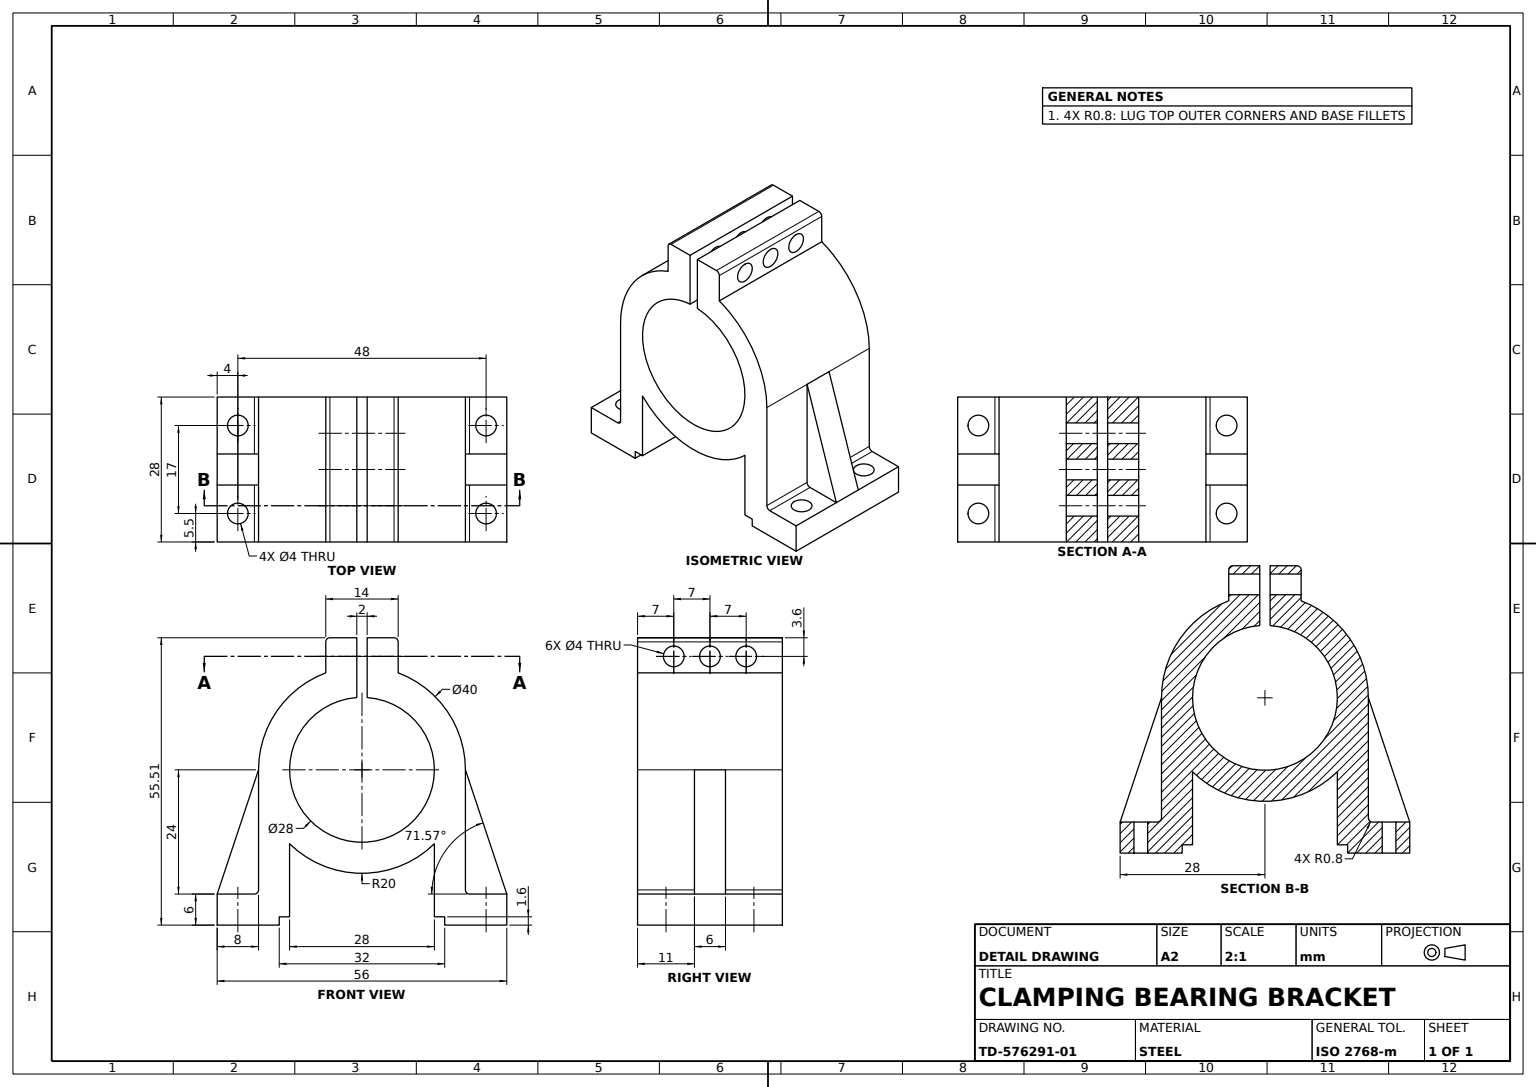
ISO-10303-21;
HEADER;
FILE_DESCRIPTION((''),'2;1');
FILE_NAME('','',(''),(''),'','','');
FILE_SCHEMA(('AUTOMOTIVE_DESIGN'));
ENDSEC;
DATA;
#1=APPLICATION_CONTEXT('');
#2=PRODUCT_CONTEXT('',#1,'mechanical');
#3=PRODUCT('','','',(#2));
#4=PRODUCT_DEFINITION_FORMATION('','',#3);
#5=PRODUCT_DEFINITION_CONTEXT('',#1,'design');
#6=PRODUCT_DEFINITION('','',#4,#5);
#7=PRODUCT_DEFINITION_SHAPE('','',#6);
#8=(LENGTH_UNIT()NAMED_UNIT(*)SI_UNIT(.MILLI.,.METRE.));
#9=(NAMED_UNIT(*)PLANE_ANGLE_UNIT()SI_UNIT($,.RADIAN.));
#10=(NAMED_UNIT(*)SI_UNIT($,.STERADIAN.)SOLID_ANGLE_UNIT());
#11=UNCERTAINTY_MEASURE_WITH_UNIT(LENGTH_MEASURE(0.005),#8,'distance_accuracy_value','');
#12=(GEOMETRIC_REPRESENTATION_CONTEXT(3)GLOBAL_UNCERTAINTY_ASSIGNED_CONTEXT((#11))GLOBAL_UNIT_ASSIGNED_CONTEXT((#8,#9,#10))REPRESENTATION_CONTEXT('',''));
#13=CARTESIAN_POINT('',(22.,-8.5,-24.));
#14=VERTEX_POINT('',#13);
#15=CARTESIAN_POINT('',(24.,-8.5,-24.));
#16=DIRECTION('',(0.,0.,-1.));
#17=DIRECTION('',(-1.,0.,0.));
#18=AXIS2_PLACEMENT_3D('',#15,#16,#17);
#19=CIRCLE('',#18,2.);
#20=EDGE_CURVE('',#14,#14,#19,.T.);
#21=ORIENTED_EDGE('',*,*,#20,.F.);
#22=EDGE_LOOP('',(#21));
#23=FACE_BOUND('',#22,.T.);
#24=CARTESIAN_POINT('',(22.,-8.5,-30.));
#25=VERTEX_POINT('',#24);
#26=CARTESIAN_POINT('',(24.,-8.5,-30.));
#27=AXIS2_PLACEMENT_3D('',#26,#16,#17);
#28=CIRCLE('',#27,2.);
#29=EDGE_CURVE('',#25,#25,#28,.T.);
#30=ORIENTED_EDGE('',*,*,#29,.T.);
#31=EDGE_LOOP('',(#30));
#32=FACE_BOUND('',#31,.T.);
#33=CYLINDRICAL_SURFACE('',#18,2.);
#34=ADVANCED_FACE('',(#23,#32),#33,.F.);
#35=CARTESIAN_POINT('',(-22.,-8.5,-30.));
#36=VERTEX_POINT('',#35);
#37=CARTESIAN_POINT('',(-24.,-8.5,-30.));
#38=DIRECTION('',(0.,0.,1.));
#39=DIRECTION('',(1.,0.,0.));
#40=AXIS2_PLACEMENT_3D('',#37,#38,#39);
#41=CIRCLE('',#40,2.);
#42=EDGE_CURVE('',#36,#36,#41,.T.);
#43=ORIENTED_EDGE('',*,*,#42,.F.);
#44=EDGE_LOOP('',(#43));
#45=FACE_BOUND('',#44,.T.);
#46=CARTESIAN_POINT('',(-26.,-8.5,-24.));
#47=VERTEX_POINT('',#46);
#48=CARTESIAN_POINT('',(-24.,-8.5,-24.));
#49=AXIS2_PLACEMENT_3D('',#48,#16,#17);
#50=CIRCLE('',#49,2.);
#51=EDGE_CURVE('',#47,#47,#50,.T.);
#52=ORIENTED_EDGE('',*,*,#51,.F.);
#53=EDGE_LOOP('',(#52));
#54=FACE_BOUND('',#53,.T.);
#55=CYLINDRICAL_SURFACE('',#49,2.);
#56=ADVANCED_FACE('',(#45,#54),#55,.F.);
#57=CARTESIAN_POINT('',(-26.,8.5,-24.));
#58=VERTEX_POINT('',#57);
#59=CARTESIAN_POINT('',(-24.,8.5,-24.));
#60=AXIS2_PLACEMENT_3D('',#59,#16,#17);
#61=CIRCLE('',#60,2.);
#62=EDGE_CURVE('',#58,#58,#61,.T.);
#63=ORIENTED_EDGE('',*,*,#62,.F.);
#64=EDGE_LOOP('',(#63));
#65=FACE_BOUND('',#64,.T.);
#66=CARTESIAN_POINT('',(-22.,8.5,-30.));
#67=VERTEX_POINT('',#66);
#68=CARTESIAN_POINT('',(-24.,8.5,-30.));
#69=AXIS2_PLACEMENT_3D('',#68,#38,#39);
#70=CIRCLE('',#69,2.);
#71=EDGE_CURVE('',#67,#67,#70,.T.);
#72=ORIENTED_EDGE('',*,*,#71,.F.);
#73=EDGE_LOOP('',(#72));
#74=FACE_BOUND('',#73,.T.);
#75=CYLINDRICAL_SURFACE('',#60,2.);
#76=ADVANCED_FACE('',(#65,#74),#75,.F.);
#77=CARTESIAN_POINT('',(22.,8.5,-30.));
#78=VERTEX_POINT('',#77);
#79=CARTESIAN_POINT('',(24.,8.5,-30.));
#80=AXIS2_PLACEMENT_3D('',#79,#16,#17);
#81=CIRCLE('',#80,2.);
#82=EDGE_CURVE('',#78,#78,#81,.T.);
#83=ORIENTED_EDGE('',*,*,#82,.T.);
#84=EDGE_LOOP('',(#83));
#85=FACE_BOUND('',#84,.T.);
#86=CARTESIAN_POINT('',(22.,8.5,-24.));
#87=VERTEX_POINT('',#86);
#88=CARTESIAN_POINT('',(24.,8.5,-24.));
#89=AXIS2_PLACEMENT_3D('',#88,#16,#17);
#90=CIRCLE('',#89,2.);
#91=EDGE_CURVE('',#87,#87,#90,.T.);
#92=ORIENTED_EDGE('',*,*,#91,.F.);
#93=EDGE_LOOP('',(#92));
#94=FACE_BOUND('',#93,.T.);
#95=CYLINDRICAL_SURFACE('',#89,2.);
#96=ADVANCED_FACE('',(#85,#94),#95,.F.);
#97=CARTESIAN_POINT('',(-7.,7.,23.914709));
#98=VERTEX_POINT('',#97);
#99=CARTESIAN_POINT('',(-7.,7.,21.914709));
#100=AXIS2_PLACEMENT_3D('',#99,#17,#38);
#101=CIRCLE('',#100,2.);
#102=EDGE_CURVE('',#98,#98,#101,.T.);
#103=ORIENTED_EDGE('',*,*,#102,.F.);
#104=EDGE_LOOP('',(#103));
#105=FACE_BOUND('',#104,.T.);
#106=CARTESIAN_POINT('',(-7.,-7.,23.914709));
#107=VERTEX_POINT('',#106);
#108=CARTESIAN_POINT('',(-7.,-7.,21.914709));
#109=AXIS2_PLACEMENT_3D('',#108,#17,#38);
#110=CIRCLE('',#109,2.);
#111=EDGE_CURVE('',#107,#107,#110,.T.);
#112=ORIENTED_EDGE('',*,*,#111,.F.);
#113=EDGE_LOOP('',(#112));
#114=FACE_BOUND('',#113,.T.);
#115=CARTESIAN_POINT('',(-7.,-14.,24.714709));
#116=VERTEX_POINT('',#115);
#117=CARTESIAN_POINT('',(-7.,14.,24.714709));
#118=VERTEX_POINT('',#117);
#119=DIRECTION('',(0.,1.,0.));
#120=VECTOR('',#119,1000.);
#121=LINE('',#115,#120);
#122=EDGE_CURVE('',#116,#118,#121,.T.);
#123=ORIENTED_EDGE('',*,*,#122,.T.);
#124=CARTESIAN_POINT('',(-7.,14.,18.734994));
#125=VERTEX_POINT('',#124);
#126=CARTESIAN_POINT('',(-7.,14.,18.314709));
#127=VECTOR('',#38,1000.);
#128=LINE('',#126,#127);
#129=EDGE_CURVE('',#125,#118,#128,.T.);
#130=ORIENTED_EDGE('',*,*,#129,.F.);
#131=CARTESIAN_POINT('',(-7.,-14.,18.734994));
#132=VERTEX_POINT('',#131);
#133=LINE('',#131,#120);
#134=EDGE_CURVE('',#132,#125,#133,.T.);
#135=ORIENTED_EDGE('',*,*,#134,.F.);
#136=CARTESIAN_POINT('',(-7.,-14.,18.314709));
#137=LINE('',#136,#127);
#138=EDGE_CURVE('',#132,#116,#137,.T.);
#139=ORIENTED_EDGE('',*,*,#138,.T.);
#140=EDGE_LOOP('',(#123,#130,#135,#139));
#141=FACE_BOUND('',#140,.T.);
#142=CARTESIAN_POINT('',(-7.,0.,23.914709));
#143=VERTEX_POINT('',#142);
#144=CARTESIAN_POINT('',(-7.,0.,21.914709));
#145=AXIS2_PLACEMENT_3D('',#144,#17,#38);
#146=CIRCLE('',#145,2.);
#147=EDGE_CURVE('',#143,#143,#146,.T.);
#148=ORIENTED_EDGE('',*,*,#147,.F.);
#149=EDGE_LOOP('',(#148));
#150=FACE_BOUND('',#149,.T.);
#151=AXIS2_PLACEMENT_3D('',#136,#17,#38);
#152=PLANE('',#151);
#153=ADVANCED_FACE('',(#105,#114,#141,#150),#152,.T.);
#154=CARTESIAN_POINT('',(20.,3.,0.));
#155=VERTEX_POINT('',#154);
#156=CARTESIAN_POINT('',(20.,3.,-23.2));
#157=VERTEX_POINT('',#156);
#158=VECTOR('',#16,1000.);
#159=LINE('',#154,#158);
#160=EDGE_CURVE('',#155,#157,#159,.T.);
#161=ORIENTED_EDGE('',*,*,#160,.F.);
#162=CARTESIAN_POINT('',(28.,3.,-24.));
#163=VERTEX_POINT('',#162);
#164=DIRECTION('',(-0.316227766,0.,0.948683298));
#165=VECTOR('',#164,1000.);
#166=LINE('',#162,#165);
#167=EDGE_CURVE('',#163,#155,#166,.T.);
#168=ORIENTED_EDGE('',*,*,#167,.F.);
#169=CARTESIAN_POINT('',(20.8,3.,-24.));
#170=VERTEX_POINT('',#169);
#171=CARTESIAN_POINT('',(20.,3.,-24.));
#172=VECTOR('',#39,1000.);
#173=LINE('',#171,#172);
#174=EDGE_CURVE('',#170,#163,#173,.T.);
#175=ORIENTED_EDGE('',*,*,#174,.F.);
#176=CARTESIAN_POINT('',(20.8,3.,-23.2));
#177=AXIS2_PLACEMENT_3D('',#176,#119,#38);
#178=CIRCLE('',#177,0.8);
#179=EDGE_CURVE('',#170,#157,#178,.T.);
#180=ORIENTED_EDGE('',*,*,#179,.T.);
#181=EDGE_LOOP('',(#161,#168,#175,#180));
#182=FACE_BOUND('',#181,.T.);
#183=CARTESIAN_POINT('',(0.,3.,0.));
#184=AXIS2_PLACEMENT_3D('',#183,#119,#38);
#185=PLANE('',#184);
#186=ADVANCED_FACE('',(#182),#185,.T.);
#187=CARTESIAN_POINT('',(-20.8,3.,-24.));
#188=VERTEX_POINT('',#187);
#189=CARTESIAN_POINT('',(-28.,3.,-24.));
#190=VERTEX_POINT('',#189);
#191=CARTESIAN_POINT('',(-20.,3.,-24.));
#192=VECTOR('',#17,1000.);
#193=LINE('',#191,#192);
#194=EDGE_CURVE('',#188,#190,#193,.T.);
#195=ORIENTED_EDGE('',*,*,#194,.F.);
#196=CARTESIAN_POINT('',(-20.8,14.,-24.));
#197=VERTEX_POINT('',#196);
#198=CARTESIAN_POINT('',(-20.8,0.,-24.));
#199=DIRECTION('',(0.,-1.,0.));
#200=VECTOR('',#199,1000.);
#201=LINE('',#198,#200);
#202=EDGE_CURVE('',#188,#197,#201,.F.);
#203=ORIENTED_EDGE('',*,*,#202,.T.);
#204=CARTESIAN_POINT('',(-28.,14.,-24.));
#205=VERTEX_POINT('',#204);
#206=CARTESIAN_POINT('',(-14.,14.,-24.));
#207=LINE('',#206,#192);
#208=EDGE_CURVE('',#197,#205,#207,.T.);
#209=ORIENTED_EDGE('',*,*,#208,.T.);
#210=LINE('',#204,#200);
#211=EDGE_CURVE('',#205,#190,#210,.T.);
#212=ORIENTED_EDGE('',*,*,#211,.T.);
#213=EDGE_LOOP('',(#195,#203,#209,#212));
#214=FACE_BOUND('',#213,.T.);
#215=ORIENTED_EDGE('',*,*,#62,.T.);
#216=EDGE_LOOP('',(#215));
#217=FACE_BOUND('',#216,.T.);
#218=CARTESIAN_POINT('',(0.,0.,-24.));
#219=AXIS2_PLACEMENT_3D('',#218,#38,#39);
#220=PLANE('',#219);
#221=ADVANCED_FACE('',(#214,#217),#220,.T.);
#222=CARTESIAN_POINT('',(-28.,14.,-30.));
#223=VERTEX_POINT('',#222);
#224=LINE('',#222,#127);
#225=EDGE_CURVE('',#223,#205,#224,.T.);
#226=ORIENTED_EDGE('',*,*,#225,.F.);
#227=CARTESIAN_POINT('',(-28.,-14.,-30.));
#228=VERTEX_POINT('',#227);
#229=LINE('',#222,#200);
#230=EDGE_CURVE('',#223,#228,#229,.T.);
#231=ORIENTED_EDGE('',*,*,#230,.T.);
#232=CARTESIAN_POINT('',(-28.,-14.,-24.));
#233=VERTEX_POINT('',#232);
#234=LINE('',#227,#127);
#235=EDGE_CURVE('',#228,#233,#234,.T.);
#236=ORIENTED_EDGE('',*,*,#235,.T.);
#237=CARTESIAN_POINT('',(-28.,-3.,-24.));
#238=VERTEX_POINT('',#237);
#239=EDGE_CURVE('',#238,#233,#210,.T.);
#240=ORIENTED_EDGE('',*,*,#239,.F.);
#241=LINE('',#237,#120);
#242=EDGE_CURVE('',#238,#190,#241,.T.);
#243=ORIENTED_EDGE('',*,*,#242,.T.);
#244=ORIENTED_EDGE('',*,*,#211,.F.);
#245=EDGE_LOOP('',(#226,#231,#236,#240,#243,#244));
#246=FACE_BOUND('',#245,.T.);
#247=AXIS2_PLACEMENT_3D('',#222,#17,#38);
#248=PLANE('',#247);
#249=ADVANCED_FACE('',(#246),#248,.T.);
#250=CARTESIAN_POINT('',(-20.,-3.,0.));
#251=VERTEX_POINT('',#250);
#252=DIRECTION('',(0.316227766,0.,0.948683298));
#253=VECTOR('',#252,1000.);
#254=LINE('',#237,#253);
#255=EDGE_CURVE('',#238,#251,#254,.T.);
#256=ORIENTED_EDGE('',*,*,#255,.T.);
#257=CARTESIAN_POINT('',(-20.,3.,0.));
#258=VERTEX_POINT('',#257);
#259=LINE('',#250,#120);
#260=EDGE_CURVE('',#251,#258,#259,.T.);
#261=ORIENTED_EDGE('',*,*,#260,.T.);
#262=LINE('',#189,#253);
#263=EDGE_CURVE('',#190,#258,#262,.T.);
#264=ORIENTED_EDGE('',*,*,#263,.F.);
#265=ORIENTED_EDGE('',*,*,#242,.F.);
#266=EDGE_LOOP('',(#256,#261,#264,#265));
#267=FACE_BOUND('',#266,.T.);
#268=DIRECTION('',(-0.948683298,0.,0.316227766));
#269=AXIS2_PLACEMENT_3D('',#237,#268,#252);
#270=PLANE('',#269);
#271=ADVANCED_FACE('',(#267),#270,.T.);
#272=CARTESIAN_POINT('',(7.,-14.,24.714709));
#273=VERTEX_POINT('',#272);
#274=CARTESIAN_POINT('',(6.2,-14.,25.514709));
#275=VERTEX_POINT('',#274);
#276=CARTESIAN_POINT('',(6.2,-14.,24.714709));
#277=AXIS2_PLACEMENT_3D('',#276,#199,#16);
#278=CIRCLE('',#277,0.8);
#279=EDGE_CURVE('',#273,#275,#278,.T.);
#280=ORIENTED_EDGE('',*,*,#279,.F.);
#281=CARTESIAN_POINT('',(7.,14.,24.714709));
#282=VERTEX_POINT('',#281);
#283=LINE('',#272,#120);
#284=EDGE_CURVE('',#282,#273,#283,.F.);
#285=ORIENTED_EDGE('',*,*,#284,.F.);
#286=CARTESIAN_POINT('',(6.2,14.,25.514709));
#287=VERTEX_POINT('',#286);
#288=CARTESIAN_POINT('',(6.2,14.,24.714709));
#289=AXIS2_PLACEMENT_3D('',#288,#199,#16);
#290=CIRCLE('',#289,0.8);
#291=EDGE_CURVE('',#287,#282,#290,.F.);
#292=ORIENTED_EDGE('',*,*,#291,.F.);
#293=LINE('',#274,#120);
#294=EDGE_CURVE('',#275,#287,#293,.T.);
#295=ORIENTED_EDGE('',*,*,#294,.F.);
#296=EDGE_LOOP('',(#280,#285,#292,#295));
#297=FACE_BOUND('',#296,.T.);
#298=AXIS2_PLACEMENT_3D('',#276,#119,#38);
#299=CYLINDRICAL_SURFACE('',#298,0.8);
#300=ADVANCED_FACE('',(#297),#299,.T.);
#301=ORIENTED_EDGE('',*,*,#82,.F.);
#302=EDGE_LOOP('',(#301));
#303=FACE_BOUND('',#302,.T.);
#304=CARTESIAN_POINT('',(16.,-14.,-30.));
#305=VERTEX_POINT('',#304);
#306=CARTESIAN_POINT('',(16.,14.,-30.));
#307=VERTEX_POINT('',#306);
#308=CARTESIAN_POINT('',(16.,-16.,-30.));
#309=LINE('',#308,#120);
#310=EDGE_CURVE('',#305,#307,#309,.T.);
#311=ORIENTED_EDGE('',*,*,#310,.T.);
#312=CARTESIAN_POINT('',(28.,14.,-30.));
#313=VERTEX_POINT('',#312);
#314=CARTESIAN_POINT('',(14.,14.,-30.));
#315=LINE('',#314,#172);
#316=EDGE_CURVE('',#307,#313,#315,.T.);
#317=ORIENTED_EDGE('',*,*,#316,.T.);
#318=CARTESIAN_POINT('',(28.,-14.,-30.));
#319=VERTEX_POINT('',#318);
#320=LINE('',#312,#200);
#321=EDGE_CURVE('',#313,#319,#320,.T.);
#322=ORIENTED_EDGE('',*,*,#321,.T.);
#323=LINE('',#318,#192);
#324=EDGE_CURVE('',#319,#305,#323,.T.);
#325=ORIENTED_EDGE('',*,*,#324,.T.);
#326=EDGE_LOOP('',(#311,#317,#322,#325));
#327=FACE_BOUND('',#326,.T.);
#328=ORIENTED_EDGE('',*,*,#29,.F.);
#329=EDGE_LOOP('',(#328));
#330=FACE_BOUND('',#329,.T.);
#331=CARTESIAN_POINT('',(0.,0.,-30.));
#332=AXIS2_PLACEMENT_3D('',#331,#16,#17);
#333=PLANE('',#332);
#334=ADVANCED_FACE('',(#303,#327,#330),#333,.T.);
#335=CARTESIAN_POINT('',(20.8,-3.,-24.));
#336=VERTEX_POINT('',#335);
#337=CARTESIAN_POINT('',(28.,-3.,-24.));
#338=VERTEX_POINT('',#337);
#339=CARTESIAN_POINT('',(20.,-3.,-24.));
#340=LINE('',#339,#172);
#341=EDGE_CURVE('',#336,#338,#340,.T.);
#342=ORIENTED_EDGE('',*,*,#341,.T.);
#343=CARTESIAN_POINT('',(20.,-3.,0.));
#344=VERTEX_POINT('',#343);
#345=LINE('',#337,#165);
#346=EDGE_CURVE('',#338,#344,#345,.T.);
#347=ORIENTED_EDGE('',*,*,#346,.T.);
#348=CARTESIAN_POINT('',(20.,-3.,-23.2));
#349=VERTEX_POINT('',#348);
#350=LINE('',#343,#158);
#351=EDGE_CURVE('',#344,#349,#350,.T.);
#352=ORIENTED_EDGE('',*,*,#351,.T.);
#353=CARTESIAN_POINT('',(20.8,-3.,-23.2));
#354=AXIS2_PLACEMENT_3D('',#353,#119,#38);
#355=CIRCLE('',#354,0.8);
#356=EDGE_CURVE('',#349,#336,#355,.F.);
#357=ORIENTED_EDGE('',*,*,#356,.T.);
#358=EDGE_LOOP('',(#342,#347,#352,#357));
#359=FACE_BOUND('',#358,.T.);
#360=CARTESIAN_POINT('',(0.,-3.,0.));
#361=AXIS2_PLACEMENT_3D('',#360,#119,#38);
#362=PLANE('',#361);
#363=ADVANCED_FACE('',(#359),#362,.F.);
#364=CARTESIAN_POINT('',(1.,7.,23.914709));
#365=VERTEX_POINT('',#364);
#366=CARTESIAN_POINT('',(1.,7.,21.914709));
#367=AXIS2_PLACEMENT_3D('',#366,#17,#38);
#368=CIRCLE('',#367,2.);
#369=EDGE_CURVE('',#365,#365,#368,.T.);
#370=ORIENTED_EDGE('',*,*,#369,.F.);
#371=EDGE_LOOP('',(#370));
#372=FACE_BOUND('',#371,.T.);
#373=CARTESIAN_POINT('',(1.,0.,23.914709));
#374=VERTEX_POINT('',#373);
#375=CARTESIAN_POINT('',(1.,0.,21.914709));
#376=AXIS2_PLACEMENT_3D('',#375,#17,#38);
#377=CIRCLE('',#376,2.);
#378=EDGE_CURVE('',#374,#374,#377,.T.);
#379=ORIENTED_EDGE('',*,*,#378,.F.);
#380=EDGE_LOOP('',(#379));
#381=FACE_BOUND('',#380,.T.);
#382=CARTESIAN_POINT('',(1.,-7.,23.914709));
#383=VERTEX_POINT('',#382);
#384=CARTESIAN_POINT('',(1.,-7.,21.914709));
#385=AXIS2_PLACEMENT_3D('',#384,#17,#38);
#386=CIRCLE('',#385,2.);
#387=EDGE_CURVE('',#383,#383,#386,.T.);
#388=ORIENTED_EDGE('',*,*,#387,.F.);
#389=EDGE_LOOP('',(#388));
#390=FACE_BOUND('',#389,.T.);
#391=CARTESIAN_POINT('',(1.,14.,25.514709));
#392=VERTEX_POINT('',#391);
#393=CARTESIAN_POINT('',(1.,-14.,25.514709));
#394=VERTEX_POINT('',#393);
#395=LINE('',#393,#200);
#396=EDGE_CURVE('',#392,#394,#395,.T.);
#397=ORIENTED_EDGE('',*,*,#396,.F.);
#398=CARTESIAN_POINT('',(1.,14.,13.96424));
#399=VERTEX_POINT('',#398);
#400=CARTESIAN_POINT('',(1.,14.,0.));
#401=LINE('',#400,#158);
#402=EDGE_CURVE('',#392,#399,#401,.T.);
#403=ORIENTED_EDGE('',*,*,#402,.T.);
#404=CARTESIAN_POINT('',(1.,-14.,13.96424));
#405=VERTEX_POINT('',#404);
#406=LINE('',#404,#120);
#407=EDGE_CURVE('',#399,#405,#406,.F.);
#408=ORIENTED_EDGE('',*,*,#407,.T.);
#409=CARTESIAN_POINT('',(1.,-14.,0.));
#410=LINE('',#409,#158);
#411=EDGE_CURVE('',#394,#405,#410,.T.);
#412=ORIENTED_EDGE('',*,*,#411,.F.);
#413=EDGE_LOOP('',(#397,#403,#408,#412));
#414=FACE_BOUND('',#413,.T.);
#415=CARTESIAN_POINT('',(1.,-17.5,12.763345));
#416=AXIS2_PLACEMENT_3D('',#415,#17,#38);
#417=PLANE('',#416);
#418=ADVANCED_FACE('',(#372,#381,#390,#414),#417,.T.);
#419=LINE('',#343,#120);
#420=EDGE_CURVE('',#344,#155,#419,.T.);
#421=ORIENTED_EDGE('',*,*,#420,.F.);
#422=ORIENTED_EDGE('',*,*,#346,.F.);
#423=LINE('',#337,#120);
#424=EDGE_CURVE('',#338,#163,#423,.T.);
#425=ORIENTED_EDGE('',*,*,#424,.T.);
#426=ORIENTED_EDGE('',*,*,#167,.T.);
#427=EDGE_LOOP('',(#421,#422,#425,#426));
#428=FACE_BOUND('',#427,.T.);
#429=DIRECTION('',(-0.948683298,0.,-0.316227766));
#430=AXIS2_PLACEMENT_3D('',#337,#429,#164);
#431=PLANE('',#430);
#432=ADVANCED_FACE('',(#428),#431,.F.);
#433=CARTESIAN_POINT('',(-6.2,14.,25.514709));
#434=VERTEX_POINT('',#433);
#435=CARTESIAN_POINT('',(-6.2,14.,24.714709));
#436=AXIS2_PLACEMENT_3D('',#435,#199,#16);
#437=CIRCLE('',#436,0.8);
#438=EDGE_CURVE('',#118,#434,#437,.F.);
#439=ORIENTED_EDGE('',*,*,#438,.F.);
#440=ORIENTED_EDGE('',*,*,#122,.F.);
#441=CARTESIAN_POINT('',(-6.2,-14.,25.514709));
#442=VERTEX_POINT('',#441);
#443=CARTESIAN_POINT('',(-6.2,-14.,24.714709));
#444=AXIS2_PLACEMENT_3D('',#443,#199,#16);
#445=CIRCLE('',#444,0.8);
#446=EDGE_CURVE('',#442,#116,#445,.T.);
#447=ORIENTED_EDGE('',*,*,#446,.F.);
#448=LINE('',#441,#120);
#449=EDGE_CURVE('',#434,#442,#448,.F.);
#450=ORIENTED_EDGE('',*,*,#449,.F.);
#451=EDGE_LOOP('',(#439,#440,#447,#450));
#452=FACE_BOUND('',#451,.T.);
#453=AXIS2_PLACEMENT_3D('',#443,#119,#38);
#454=CYLINDRICAL_SURFACE('',#453,0.8);
#455=ADVANCED_FACE('',(#452),#454,.T.);
#456=ORIENTED_EDGE('',*,*,#20,.T.);
#457=EDGE_LOOP('',(#456));
#458=FACE_BOUND('',#457,.T.);
#459=ORIENTED_EDGE('',*,*,#341,.F.);
#460=CARTESIAN_POINT('',(20.8,-14.,-24.));
#461=VERTEX_POINT('',#460);
#462=LINE('',#460,#200);
#463=EDGE_CURVE('',#336,#461,#462,.T.);
#464=ORIENTED_EDGE('',*,*,#463,.T.);
#465=CARTESIAN_POINT('',(28.,-14.,-24.));
#466=VERTEX_POINT('',#465);
#467=LINE('',#465,#192);
#468=EDGE_CURVE('',#466,#461,#467,.T.);
#469=ORIENTED_EDGE('',*,*,#468,.F.);
#470=CARTESIAN_POINT('',(28.,14.,-24.));
#471=LINE('',#470,#200);
#472=EDGE_CURVE('',#338,#466,#471,.T.);
#473=ORIENTED_EDGE('',*,*,#472,.F.);
#474=EDGE_LOOP('',(#459,#464,#469,#473));
#475=FACE_BOUND('',#474,.T.);
#476=AXIS2_PLACEMENT_3D('',#218,#16,#17);
#477=PLANE('',#476);
#478=ADVANCED_FACE('',(#458,#475),#477,.F.);
#479=CARTESIAN_POINT('',(-1.,0.,19.914709));
#480=VERTEX_POINT('',#479);
#481=CARTESIAN_POINT('',(-1.,0.,21.914709));
#482=AXIS2_PLACEMENT_3D('',#481,#39,#16);
#483=CIRCLE('',#482,2.);
#484=EDGE_CURVE('',#480,#480,#483,.T.);
#485=ORIENTED_EDGE('',*,*,#484,.T.);
#486=EDGE_LOOP('',(#485));
#487=FACE_BOUND('',#486,.T.);
#488=ORIENTED_EDGE('',*,*,#147,.T.);
#489=EDGE_LOOP('',(#488));
#490=FACE_BOUND('',#489,.T.);
#491=CARTESIAN_POINT('',(7.,0.,21.914709));
#492=AXIS2_PLACEMENT_3D('',#491,#17,#38);
#493=CYLINDRICAL_SURFACE('',#492,2.);
#494=ADVANCED_FACE('',(#487,#490),#493,.F.);
#495=CARTESIAN_POINT('',(-20.,14.,0.));
#496=VERTEX_POINT('',#495);
#497=CARTESIAN_POINT('',(-20.,14.,-23.2));
#498=VERTEX_POINT('',#497);
#499=LINE('',#495,#158);
#500=EDGE_CURVE('',#496,#498,#499,.T.);
#501=ORIENTED_EDGE('',*,*,#500,.F.);
#502=CARTESIAN_POINT('',(0.,14.,0.));
#503=AXIS2_PLACEMENT_3D('',#502,#199,#39);
#504=CIRCLE('',#503,20.);
#505=EDGE_CURVE('',#125,#496,#504,.T.);
#506=ORIENTED_EDGE('',*,*,#505,.F.);
#507=ORIENTED_EDGE('',*,*,#129,.T.);
#508=ORIENTED_EDGE('',*,*,#438,.T.);
#509=CARTESIAN_POINT('',(-1.,14.,25.514709));
#510=VERTEX_POINT('',#509);
#511=CARTESIAN_POINT('',(-7.,14.,25.514709));
#512=LINE('',#511,#172);
#513=EDGE_CURVE('',#434,#510,#512,.T.);
#514=ORIENTED_EDGE('',*,*,#513,.T.);
#515=CARTESIAN_POINT('',(-1.,14.,13.96424));
#516=VERTEX_POINT('',#515);
#517=CARTESIAN_POINT('',(-1.,14.,0.));
#518=LINE('',#517,#127);
#519=EDGE_CURVE('',#516,#510,#518,.T.);
#520=ORIENTED_EDGE('',*,*,#519,.F.);
#521=AXIS2_PLACEMENT_3D('',#502,#199,#16);
#522=CIRCLE('',#521,14.);
#523=EDGE_CURVE('',#516,#399,#522,.T.);
#524=ORIENTED_EDGE('',*,*,#523,.T.);
#525=ORIENTED_EDGE('',*,*,#402,.F.);
#526=EDGE_CURVE('',#392,#287,#512,.T.);
#527=ORIENTED_EDGE('',*,*,#526,.T.);
#528=ORIENTED_EDGE('',*,*,#291,.T.);
#529=CARTESIAN_POINT('',(7.,14.,18.734994));
#530=VERTEX_POINT('',#529);
#531=CARTESIAN_POINT('',(7.,14.,25.514709));
#532=LINE('',#531,#158);
#533=EDGE_CURVE('',#282,#530,#532,.T.);
#534=ORIENTED_EDGE('',*,*,#533,.T.);
#535=CARTESIAN_POINT('',(20.,14.,0.));
#536=VERTEX_POINT('',#535);
#537=EDGE_CURVE('',#536,#530,#504,.T.);
#538=ORIENTED_EDGE('',*,*,#537,.F.);
#539=CARTESIAN_POINT('',(20.,14.,-23.2));
#540=VERTEX_POINT('',#539);
#541=CARTESIAN_POINT('',(20.,14.,-24.));
#542=LINE('',#541,#127);
#543=EDGE_CURVE('',#540,#536,#542,.T.);
#544=ORIENTED_EDGE('',*,*,#543,.F.);
#545=CARTESIAN_POINT('',(20.8,14.,-24.));
#546=VERTEX_POINT('',#545);
#547=CARTESIAN_POINT('',(20.8,14.,-23.2));
#548=AXIS2_PLACEMENT_3D('',#547,#199,#16);
#549=CIRCLE('',#548,0.8);
#550=EDGE_CURVE('',#540,#546,#549,.T.);
#551=ORIENTED_EDGE('',*,*,#550,.T.);
#552=VERTEX_POINT('',#470);
#553=CARTESIAN_POINT('',(14.,14.,-24.));
#554=LINE('',#553,#172);
#555=EDGE_CURVE('',#546,#552,#554,.T.);
#556=ORIENTED_EDGE('',*,*,#555,.T.);
#557=LINE('',#312,#127);
#558=EDGE_CURVE('',#313,#552,#557,.T.);
#559=ORIENTED_EDGE('',*,*,#558,.F.);
#560=ORIENTED_EDGE('',*,*,#316,.F.);
#561=CARTESIAN_POINT('',(16.,14.,-28.4));
#562=VERTEX_POINT('',#561);
#563=CARTESIAN_POINT('',(16.,14.,0.));
#564=LINE('',#563,#127);
#565=EDGE_CURVE('',#307,#562,#564,.T.);
#566=ORIENTED_EDGE('',*,*,#565,.T.);
#567=CARTESIAN_POINT('',(14.,14.,-28.4));
#568=VERTEX_POINT('',#567);
#569=CARTESIAN_POINT('',(0.,14.,-28.4));
#570=LINE('',#569,#192);
#571=EDGE_CURVE('',#562,#568,#570,.T.);
#572=ORIENTED_EDGE('',*,*,#571,.T.);
#573=CARTESIAN_POINT('',(14.,14.,-14.282857));
#574=VERTEX_POINT('',#573);
#575=CARTESIAN_POINT('',(14.,14.,0.));
#576=LINE('',#575,#158);
#577=EDGE_CURVE('',#574,#568,#576,.T.);
#578=ORIENTED_EDGE('',*,*,#577,.F.);
#579=CARTESIAN_POINT('',(-14.,14.,-14.282857));
#580=VERTEX_POINT('',#579);
#581=CIRCLE('',#521,20.);
#582=EDGE_CURVE('',#580,#574,#581,.T.);
#583=ORIENTED_EDGE('',*,*,#582,.F.);
#584=CARTESIAN_POINT('',(-14.,14.,-28.4));
#585=VERTEX_POINT('',#584);
#586=CARTESIAN_POINT('',(-14.,14.,0.));
#587=LINE('',#586,#127);
#588=EDGE_CURVE('',#585,#580,#587,.T.);
#589=ORIENTED_EDGE('',*,*,#588,.F.);
#590=CARTESIAN_POINT('',(-16.,14.,-28.4));
#591=VERTEX_POINT('',#590);
#592=LINE('',#569,#172);
#593=EDGE_CURVE('',#591,#585,#592,.T.);
#594=ORIENTED_EDGE('',*,*,#593,.F.);
#595=CARTESIAN_POINT('',(-16.,14.,-30.));
#596=VERTEX_POINT('',#595);
#597=CARTESIAN_POINT('',(-16.,14.,0.));
#598=LINE('',#597,#127);
#599=EDGE_CURVE('',#596,#591,#598,.T.);
#600=ORIENTED_EDGE('',*,*,#599,.F.);
#601=CARTESIAN_POINT('',(-14.,14.,-30.));
#602=LINE('',#601,#192);
#603=EDGE_CURVE('',#596,#223,#602,.T.);
#604=ORIENTED_EDGE('',*,*,#603,.T.);
#605=ORIENTED_EDGE('',*,*,#225,.T.);
#606=ORIENTED_EDGE('',*,*,#208,.F.);
#607=CARTESIAN_POINT('',(-20.8,14.,-23.2));
#608=AXIS2_PLACEMENT_3D('',#607,#199,#16);
#609=CIRCLE('',#608,0.8);
#610=EDGE_CURVE('',#197,#498,#609,.T.);
#611=ORIENTED_EDGE('',*,*,#610,.T.);
#612=EDGE_LOOP('',(#501,#506,#507,#508,#514,#520,#524,#525,#527,#528,#534,#538,#544,#551,#556,#559,#560,#566,#572,#578,#583,#589,#594,#600,#604,#605,#606,#611));
#613=FACE_BOUND('',#612,.T.);
#614=PLANE('',#521);
#615=ADVANCED_FACE('',(#613),#614,.F.);
#616=ORIENTED_EDGE('',*,*,#42,.T.);
#617=EDGE_LOOP('',(#616));
#618=FACE_BOUND('',#617,.T.);
#619=ORIENTED_EDGE('',*,*,#230,.F.);
#620=ORIENTED_EDGE('',*,*,#603,.F.);
#621=CARTESIAN_POINT('',(-16.,-14.,-30.));
#622=VERTEX_POINT('',#621);
#623=CARTESIAN_POINT('',(-16.,-16.,-30.));
#624=LINE('',#623,#120);
#625=EDGE_CURVE('',#622,#596,#624,.T.);
#626=ORIENTED_EDGE('',*,*,#625,.F.);
#627=LINE('',#227,#172);
#628=EDGE_CURVE('',#228,#622,#627,.T.);
#629=ORIENTED_EDGE('',*,*,#628,.F.);
#630=EDGE_LOOP('',(#619,#620,#626,#629));
#631=FACE_BOUND('',#630,.T.);
#632=ORIENTED_EDGE('',*,*,#71,.T.);
#633=EDGE_LOOP('',(#632));
#634=FACE_BOUND('',#633,.T.);
#635=AXIS2_PLACEMENT_3D('',#331,#38,#39);
#636=PLANE('',#635);
#637=ADVANCED_FACE('',(#618,#631,#634),#636,.F.);
#638=CARTESIAN_POINT('',(-1.,-7.,19.914709));
#639=VERTEX_POINT('',#638);
#640=CARTESIAN_POINT('',(-1.,-7.,21.914709));
#641=AXIS2_PLACEMENT_3D('',#640,#39,#16);
#642=CIRCLE('',#641,2.);
#643=EDGE_CURVE('',#639,#639,#642,.T.);
#644=ORIENTED_EDGE('',*,*,#643,.F.);
#645=EDGE_LOOP('',(#644));
#646=FACE_BOUND('',#645,.T.);
#647=ORIENTED_EDGE('',*,*,#519,.T.);
#648=CARTESIAN_POINT('',(-1.,-14.,25.514709));
#649=VERTEX_POINT('',#648);
#650=LINE('',#648,#120);
#651=EDGE_CURVE('',#649,#510,#650,.T.);
#652=ORIENTED_EDGE('',*,*,#651,.F.);
#653=CARTESIAN_POINT('',(-1.,-14.,13.96424));
#654=VERTEX_POINT('',#653);
#655=CARTESIAN_POINT('',(-1.,-14.,0.));
#656=LINE('',#655,#127);
#657=EDGE_CURVE('',#654,#649,#656,.T.);
#658=ORIENTED_EDGE('',*,*,#657,.F.);
#659=LINE('',#653,#120);
#660=EDGE_CURVE('',#654,#516,#659,.T.);
#661=ORIENTED_EDGE('',*,*,#660,.T.);
#662=EDGE_LOOP('',(#647,#652,#658,#661));
#663=FACE_BOUND('',#662,.T.);
#664=ORIENTED_EDGE('',*,*,#484,.F.);
#665=EDGE_LOOP('',(#664));
#666=FACE_BOUND('',#665,.T.);
#667=CARTESIAN_POINT('',(-1.,7.,19.914709));
#668=VERTEX_POINT('',#667);
#669=CARTESIAN_POINT('',(-1.,7.,21.914709));
#670=AXIS2_PLACEMENT_3D('',#669,#39,#16);
#671=CIRCLE('',#670,2.);
#672=EDGE_CURVE('',#668,#668,#671,.T.);
#673=ORIENTED_EDGE('',*,*,#672,.F.);
#674=EDGE_LOOP('',(#673));
#675=FACE_BOUND('',#674,.T.);
#676=CARTESIAN_POINT('',(-1.,-17.5,29.202472));
#677=AXIS2_PLACEMENT_3D('',#676,#39,#16);
#678=PLANE('',#677);
#679=ADVANCED_FACE('',(#646,#663,#666,#675),#678,.T.);
#680=ORIENTED_EDGE('',*,*,#138,.F.);
#681=CARTESIAN_POINT('',(-20.,-14.,0.));
#682=VERTEX_POINT('',#681);
#683=CARTESIAN_POINT('',(0.,-14.,0.));
#684=AXIS2_PLACEMENT_3D('',#683,#199,#39);
#685=CIRCLE('',#684,20.);
#686=EDGE_CURVE('',#132,#682,#685,.T.);
#687=ORIENTED_EDGE('',*,*,#686,.T.);
#688=CARTESIAN_POINT('',(-20.,-14.,-23.2));
#689=VERTEX_POINT('',#688);
#690=LINE('',#681,#158);
#691=EDGE_CURVE('',#682,#689,#690,.T.);
#692=ORIENTED_EDGE('',*,*,#691,.T.);
#693=CARTESIAN_POINT('',(-20.8,-14.,-24.));
#694=VERTEX_POINT('',#693);
#695=CARTESIAN_POINT('',(-20.8,-14.,-23.2));
#696=AXIS2_PLACEMENT_3D('',#695,#199,#16);
#697=CIRCLE('',#696,0.8);
#698=EDGE_CURVE('',#689,#694,#697,.F.);
#699=ORIENTED_EDGE('',*,*,#698,.T.);
#700=LINE('',#232,#172);
#701=EDGE_CURVE('',#233,#694,#700,.T.);
#702=ORIENTED_EDGE('',*,*,#701,.F.);
#703=ORIENTED_EDGE('',*,*,#235,.F.);
#704=ORIENTED_EDGE('',*,*,#628,.T.);
#705=CARTESIAN_POINT('',(-16.,-14.,-28.4));
#706=VERTEX_POINT('',#705);
#707=CARTESIAN_POINT('',(-16.,-14.,0.));
#708=LINE('',#707,#127);
#709=EDGE_CURVE('',#622,#706,#708,.T.);
#710=ORIENTED_EDGE('',*,*,#709,.T.);
#711=CARTESIAN_POINT('',(-14.,-14.,-28.4));
#712=VERTEX_POINT('',#711);
#713=CARTESIAN_POINT('',(0.,-14.,-28.4));
#714=LINE('',#713,#172);
#715=EDGE_CURVE('',#706,#712,#714,.T.);
#716=ORIENTED_EDGE('',*,*,#715,.T.);
#717=CARTESIAN_POINT('',(-14.,-14.,-14.282857));
#718=VERTEX_POINT('',#717);
#719=CARTESIAN_POINT('',(-14.,-14.,0.));
#720=LINE('',#719,#127);
#721=EDGE_CURVE('',#712,#718,#720,.T.);
#722=ORIENTED_EDGE('',*,*,#721,.T.);
#723=CARTESIAN_POINT('',(14.,-14.,-14.282857));
#724=VERTEX_POINT('',#723);
#725=AXIS2_PLACEMENT_3D('',#683,#199,#16);
#726=CIRCLE('',#725,20.);
#727=EDGE_CURVE('',#718,#724,#726,.T.);
#728=ORIENTED_EDGE('',*,*,#727,.T.);
#729=CARTESIAN_POINT('',(14.,-14.,-28.4));
#730=VERTEX_POINT('',#729);
#731=CARTESIAN_POINT('',(14.,-14.,0.));
#732=LINE('',#731,#158);
#733=EDGE_CURVE('',#724,#730,#732,.T.);
#734=ORIENTED_EDGE('',*,*,#733,.T.);
#735=CARTESIAN_POINT('',(16.,-14.,-28.4));
#736=VERTEX_POINT('',#735);
#737=LINE('',#713,#192);
#738=EDGE_CURVE('',#736,#730,#737,.T.);
#739=ORIENTED_EDGE('',*,*,#738,.F.);
#740=CARTESIAN_POINT('',(16.,-14.,0.));
#741=LINE('',#740,#127);
#742=EDGE_CURVE('',#305,#736,#741,.T.);
#743=ORIENTED_EDGE('',*,*,#742,.F.);
#744=ORIENTED_EDGE('',*,*,#324,.F.);
#745=LINE('',#318,#127);
#746=EDGE_CURVE('',#319,#466,#745,.T.);
#747=ORIENTED_EDGE('',*,*,#746,.T.);
#748=ORIENTED_EDGE('',*,*,#468,.T.);
#749=CARTESIAN_POINT('',(20.,-14.,-23.2));
#750=VERTEX_POINT('',#749);
#751=CARTESIAN_POINT('',(20.8,-14.,-23.2));
#752=AXIS2_PLACEMENT_3D('',#751,#199,#16);
#753=CIRCLE('',#752,0.8);
#754=EDGE_CURVE('',#461,#750,#753,.F.);
#755=ORIENTED_EDGE('',*,*,#754,.T.);
#756=CARTESIAN_POINT('',(20.,-14.,0.));
#757=VERTEX_POINT('',#756);
#758=CARTESIAN_POINT('',(20.,-14.,-24.));
#759=LINE('',#758,#127);
#760=EDGE_CURVE('',#750,#757,#759,.T.);
#761=ORIENTED_EDGE('',*,*,#760,.T.);
#762=CARTESIAN_POINT('',(7.,-14.,18.734994));
#763=VERTEX_POINT('',#762);
#764=EDGE_CURVE('',#757,#763,#685,.T.);
#765=ORIENTED_EDGE('',*,*,#764,.T.);
#766=CARTESIAN_POINT('',(7.,-14.,25.514709));
#767=LINE('',#766,#158);
#768=EDGE_CURVE('',#273,#763,#767,.T.);
#769=ORIENTED_EDGE('',*,*,#768,.F.);
#770=ORIENTED_EDGE('',*,*,#279,.T.);
#771=CARTESIAN_POINT('',(-7.,-14.,25.514709));
#772=LINE('',#771,#172);
#773=EDGE_CURVE('',#394,#275,#772,.T.);
#774=ORIENTED_EDGE('',*,*,#773,.F.);
#775=ORIENTED_EDGE('',*,*,#411,.T.);
#776=AXIS2_PLACEMENT_3D('',#683,#119,#38);
#777=CIRCLE('',#776,14.);
#778=EDGE_CURVE('',#405,#654,#777,.T.);
#779=ORIENTED_EDGE('',*,*,#778,.T.);
#780=ORIENTED_EDGE('',*,*,#657,.T.);
#781=EDGE_CURVE('',#442,#649,#772,.T.);
#782=ORIENTED_EDGE('',*,*,#781,.F.);
#783=ORIENTED_EDGE('',*,*,#446,.T.);
#784=EDGE_LOOP('',(#680,#687,#692,#699,#702,#703,#704,#710,#716,#722,#728,#734,#739,#743,#744,#747,#748,#755,#761,#765,#769,#770,#774,#775,#779,#780,#782,#783));
#785=FACE_BOUND('',#784,.T.);
#786=PLANE('',#725);
#787=ADVANCED_FACE('',(#785),#786,.T.);
#788=CARTESIAN_POINT('',(7.,7.,23.914709));
#789=VERTEX_POINT('',#788);
#790=CARTESIAN_POINT('',(7.,7.,21.914709));
#791=AXIS2_PLACEMENT_3D('',#790,#17,#38);
#792=CIRCLE('',#791,2.);
#793=EDGE_CURVE('',#789,#789,#792,.T.);
#794=ORIENTED_EDGE('',*,*,#793,.F.);
#795=EDGE_LOOP('',(#794));
#796=FACE_BOUND('',#795,.T.);
#797=ORIENTED_EDGE('',*,*,#369,.T.);
#798=EDGE_LOOP('',(#797));
#799=FACE_BOUND('',#798,.T.);
#800=CYLINDRICAL_SURFACE('',#791,2.);
#801=ADVANCED_FACE('',(#796,#799),#800,.F.);
#802=CARTESIAN_POINT('',(14.,-21.,-14.282857));
#803=LINE('',#802,#120);
#804=EDGE_CURVE('',#574,#724,#803,.F.);
#805=ORIENTED_EDGE('',*,*,#804,.F.);
#806=ORIENTED_EDGE('',*,*,#577,.T.);
#807=CARTESIAN_POINT('',(14.,-21.,-28.4));
#808=LINE('',#807,#120);
#809=EDGE_CURVE('',#730,#568,#808,.T.);
#810=ORIENTED_EDGE('',*,*,#809,.F.);
#811=ORIENTED_EDGE('',*,*,#733,.F.);
#812=EDGE_LOOP('',(#805,#806,#810,#811));
#813=FACE_BOUND('',#812,.T.);
#814=CARTESIAN_POINT('',(14.,-21.,-30.));
#815=AXIS2_PLACEMENT_3D('',#814,#17,#38);
#816=PLANE('',#815);
#817=ADVANCED_FACE('',(#813),#816,.T.);
#818=ORIENTED_EDGE('',*,*,#294,.T.);
#819=ORIENTED_EDGE('',*,*,#526,.F.);
#820=ORIENTED_EDGE('',*,*,#396,.T.);
#821=ORIENTED_EDGE('',*,*,#773,.T.);
#822=EDGE_LOOP('',(#818,#819,#820,#821));
#823=FACE_BOUND('',#822,.T.);
#824=AXIS2_PLACEMENT_3D('',#771,#38,#39);
#825=PLANE('',#824);
#826=ADVANCED_FACE('',(#823),#825,.T.);
#827=LINE('',#348,#200);
#828=EDGE_CURVE('',#750,#349,#827,.F.);
#829=ORIENTED_EDGE('',*,*,#828,.F.);
#830=ORIENTED_EDGE('',*,*,#754,.F.);
#831=ORIENTED_EDGE('',*,*,#463,.F.);
#832=ORIENTED_EDGE('',*,*,#356,.F.);
#833=EDGE_LOOP('',(#829,#830,#831,#832));
#834=FACE_BOUND('',#833,.T.);
#835=CARTESIAN_POINT('',(20.8,0.,-23.2));
#836=AXIS2_PLACEMENT_3D('',#835,#119,#38);
#837=CYLINDRICAL_SURFACE('',#836,0.8);
#838=ADVANCED_FACE('',(#834),#837,.F.);
#839=ORIENTED_EDGE('',*,*,#809,.T.);
#840=ORIENTED_EDGE('',*,*,#571,.F.);
#841=CARTESIAN_POINT('',(16.,-16.,-28.4));
#842=LINE('',#841,#120);
#843=EDGE_CURVE('',#562,#736,#842,.F.);
#844=ORIENTED_EDGE('',*,*,#843,.T.);
#845=ORIENTED_EDGE('',*,*,#738,.T.);
#846=EDGE_LOOP('',(#839,#840,#844,#845));
#847=FACE_BOUND('',#846,.T.);
#848=CARTESIAN_POINT('',(12.,-16.,-28.4));
#849=AXIS2_PLACEMENT_3D('',#848,#38,#39);
#850=PLANE('',#849);
#851=ADVANCED_FACE('',(#847),#850,.F.);
#852=CARTESIAN_POINT('',(-20.,3.,-23.2));
#853=VERTEX_POINT('',#852);
#854=CARTESIAN_POINT('',(-20.8,3.,-23.2));
#855=AXIS2_PLACEMENT_3D('',#854,#199,#16);
#856=CIRCLE('',#855,0.8);
#857=EDGE_CURVE('',#853,#188,#856,.F.);
#858=ORIENTED_EDGE('',*,*,#857,.F.);
#859=LINE('',#688,#200);
#860=EDGE_CURVE('',#498,#853,#859,.T.);
#861=ORIENTED_EDGE('',*,*,#860,.F.);
#862=ORIENTED_EDGE('',*,*,#610,.F.);
#863=ORIENTED_EDGE('',*,*,#202,.F.);
#864=EDGE_LOOP('',(#858,#861,#862,#863));
#865=FACE_BOUND('',#864,.T.);
#866=CYLINDRICAL_SURFACE('',#696,0.8);
#867=ADVANCED_FACE('',(#865),#866,.F.);
#868=CARTESIAN_POINT('',(-20.,-3.,-23.2));
#869=VERTEX_POINT('',#868);
#870=LINE('',#250,#158);
#871=EDGE_CURVE('',#251,#869,#870,.T.);
#872=ORIENTED_EDGE('',*,*,#871,.T.);
#873=EDGE_CURVE('',#869,#689,#859,.T.);
#874=ORIENTED_EDGE('',*,*,#873,.T.);
#875=ORIENTED_EDGE('',*,*,#691,.F.);
#876=LINE('',#681,#120);
#877=EDGE_CURVE('',#682,#251,#876,.T.);
#878=ORIENTED_EDGE('',*,*,#877,.T.);
#879=EDGE_LOOP('',(#872,#874,#875,#878));
#880=FACE_BOUND('',#879,.T.);
#881=AXIS2_PLACEMENT_3D('',#681,#39,#16);
#882=PLANE('',#881);
#883=ADVANCED_FACE('',(#880),#882,.F.);
#884=ORIENTED_EDGE('',*,*,#387,.T.);
#885=EDGE_LOOP('',(#884));
#886=FACE_BOUND('',#885,.T.);
#887=CARTESIAN_POINT('',(7.,-7.,23.914709));
#888=VERTEX_POINT('',#887);
#889=CARTESIAN_POINT('',(7.,-7.,21.914709));
#890=AXIS2_PLACEMENT_3D('',#889,#17,#38);
#891=CIRCLE('',#890,2.);
#892=EDGE_CURVE('',#888,#888,#891,.T.);
#893=ORIENTED_EDGE('',*,*,#892,.F.);
#894=EDGE_LOOP('',(#893));
#895=FACE_BOUND('',#894,.T.);
#896=CYLINDRICAL_SURFACE('',#890,2.);
#897=ADVANCED_FACE('',(#886,#895),#896,.F.);
#898=ORIENTED_EDGE('',*,*,#505,.T.);
#899=EDGE_CURVE('',#258,#496,#876,.T.);
#900=ORIENTED_EDGE('',*,*,#899,.F.);
#901=ORIENTED_EDGE('',*,*,#260,.F.);
#902=ORIENTED_EDGE('',*,*,#877,.F.);
#903=ORIENTED_EDGE('',*,*,#686,.F.);
#904=ORIENTED_EDGE('',*,*,#134,.T.);
#905=EDGE_LOOP('',(#898,#900,#901,#902,#903,#904));
#906=FACE_BOUND('',#905,.T.);
#907=CYLINDRICAL_SURFACE('',#776,20.);
#908=ADVANCED_FACE('',(#906),#907,.T.);
#909=ORIENTED_EDGE('',*,*,#715,.F.);
#910=CARTESIAN_POINT('',(-16.,-16.,-28.4));
#911=LINE('',#910,#120);
#912=EDGE_CURVE('',#591,#706,#911,.F.);
#913=ORIENTED_EDGE('',*,*,#912,.F.);
#914=ORIENTED_EDGE('',*,*,#593,.T.);
#915=CARTESIAN_POINT('',(-14.,-21.,-28.4));
#916=LINE('',#915,#120);
#917=EDGE_CURVE('',#712,#585,#916,.T.);
#918=ORIENTED_EDGE('',*,*,#917,.F.);
#919=EDGE_LOOP('',(#909,#913,#914,#918));
#920=FACE_BOUND('',#919,.T.);
#921=CARTESIAN_POINT('',(-12.,-16.,-28.4));
#922=AXIS2_PLACEMENT_3D('',#921,#16,#17);
#923=PLANE('',#922);
#924=ADVANCED_FACE('',(#920),#923,.T.);
#925=ORIENTED_EDGE('',*,*,#721,.F.);
#926=ORIENTED_EDGE('',*,*,#917,.T.);
#927=ORIENTED_EDGE('',*,*,#588,.T.);
#928=CARTESIAN_POINT('',(-14.,-21.,-14.282857));
#929=LINE('',#928,#120);
#930=EDGE_CURVE('',#580,#718,#929,.F.);
#931=ORIENTED_EDGE('',*,*,#930,.T.);
#932=EDGE_LOOP('',(#925,#926,#927,#931));
#933=FACE_BOUND('',#932,.T.);
#934=AXIS2_PLACEMENT_3D('',#928,#39,#16);
#935=PLANE('',#934);
#936=ADVANCED_FACE('',(#933),#935,.T.);
#937=CARTESIAN_POINT('',(7.,0.,23.914709));
#938=VERTEX_POINT('',#937);
#939=CIRCLE('',#492,2.);
#940=EDGE_CURVE('',#938,#938,#939,.T.);
#941=ORIENTED_EDGE('',*,*,#940,.T.);
#942=EDGE_LOOP('',(#941));
#943=FACE_BOUND('',#942,.T.);
#944=ORIENTED_EDGE('',*,*,#892,.T.);
#945=EDGE_LOOP('',(#944));
#946=FACE_BOUND('',#945,.T.);
#947=ORIENTED_EDGE('',*,*,#768,.T.);
#948=LINE('',#762,#120);
#949=EDGE_CURVE('',#530,#763,#948,.F.);
#950=ORIENTED_EDGE('',*,*,#949,.F.);
#951=ORIENTED_EDGE('',*,*,#533,.F.);
#952=ORIENTED_EDGE('',*,*,#284,.T.);
#953=EDGE_LOOP('',(#947,#950,#951,#952));
#954=FACE_BOUND('',#953,.T.);
#955=ORIENTED_EDGE('',*,*,#793,.T.);
#956=EDGE_LOOP('',(#955));
#957=FACE_BOUND('',#956,.T.);
#958=AXIS2_PLACEMENT_3D('',#766,#39,#16);
#959=PLANE('',#958);
#960=ADVANCED_FACE('',(#943,#946,#954,#957),#959,.T.);
#961=ORIENTED_EDGE('',*,*,#930,.F.);
#962=ORIENTED_EDGE('',*,*,#582,.T.);
#963=ORIENTED_EDGE('',*,*,#804,.T.);
#964=ORIENTED_EDGE('',*,*,#727,.F.);
#965=EDGE_LOOP('',(#961,#962,#963,#964));
#966=FACE_BOUND('',#965,.T.);
#967=CARTESIAN_POINT('',(0.,-21.,0.));
#968=AXIS2_PLACEMENT_3D('',#967,#119,#38);
#969=CYLINDRICAL_SURFACE('',#968,20.);
#970=ADVANCED_FACE('',(#966),#969,.T.);
#971=ORIENTED_EDGE('',*,*,#778,.F.);
#972=ORIENTED_EDGE('',*,*,#407,.F.);
#973=ORIENTED_EDGE('',*,*,#523,.F.);
#974=ORIENTED_EDGE('',*,*,#660,.F.);
#975=EDGE_LOOP('',(#971,#972,#973,#974));
#976=FACE_BOUND('',#975,.T.);
#977=CYLINDRICAL_SURFACE('',#776,14.);
#978=ADVANCED_FACE('',(#976),#977,.F.);
#979=ORIENTED_EDGE('',*,*,#828,.T.);
#980=ORIENTED_EDGE('',*,*,#351,.F.);
#981=LINE('',#756,#120);
#982=EDGE_CURVE('',#757,#344,#981,.T.);
#983=ORIENTED_EDGE('',*,*,#982,.F.);
#984=ORIENTED_EDGE('',*,*,#760,.F.);
#985=EDGE_LOOP('',(#979,#980,#983,#984));
#986=FACE_BOUND('',#985,.T.);
#987=AXIS2_PLACEMENT_3D('',#758,#17,#38);
#988=PLANE('',#987);
#989=ADVANCED_FACE('',(#986),#988,.F.);
#990=ORIENTED_EDGE('',*,*,#742,.T.);
#991=ORIENTED_EDGE('',*,*,#843,.F.);
#992=ORIENTED_EDGE('',*,*,#565,.F.);
#993=ORIENTED_EDGE('',*,*,#310,.F.);
#994=EDGE_LOOP('',(#990,#991,#992,#993));
#995=FACE_BOUND('',#994,.T.);
#996=AXIS2_PLACEMENT_3D('',#841,#39,#16);
#997=PLANE('',#996);
#998=ADVANCED_FACE('',(#995),#997,.F.);
#999=CARTESIAN_POINT('',(-20.8,-3.,-24.));
#1000=VERTEX_POINT('',#999);
#1001=CARTESIAN_POINT('',(-20.,-3.,-24.));
#1002=LINE('',#1001,#192);
#1003=EDGE_CURVE('',#1000,#238,#1002,.T.);
#1004=ORIENTED_EDGE('',*,*,#1003,.F.);
#1005=CARTESIAN_POINT('',(-20.8,-3.,-23.2));
#1006=AXIS2_PLACEMENT_3D('',#1005,#199,#16);
#1007=CIRCLE('',#1006,0.8);
#1008=EDGE_CURVE('',#1000,#869,#1007,.T.);
#1009=ORIENTED_EDGE('',*,*,#1008,.T.);
#1010=ORIENTED_EDGE('',*,*,#871,.F.);
#1011=ORIENTED_EDGE('',*,*,#255,.F.);
#1012=EDGE_LOOP('',(#1004,#1009,#1010,#1011));
#1013=FACE_BOUND('',#1012,.T.);
#1014=AXIS2_PLACEMENT_3D('',#360,#199,#16);
#1015=PLANE('',#1014);
#1016=ADVANCED_FACE('',(#1013),#1015,.T.);
#1017=ORIENTED_EDGE('',*,*,#912,.T.);
#1018=ORIENTED_EDGE('',*,*,#709,.F.);
#1019=ORIENTED_EDGE('',*,*,#625,.T.);
#1020=ORIENTED_EDGE('',*,*,#599,.T.);
#1021=EDGE_LOOP('',(#1017,#1018,#1019,#1020));
#1022=FACE_BOUND('',#1021,.T.);
#1023=AXIS2_PLACEMENT_3D('',#910,#39,#16);
#1024=PLANE('',#1023);
#1025=ADVANCED_FACE('',(#1022),#1024,.T.);
#1026=ORIENTED_EDGE('',*,*,#543,.T.);
#1027=EDGE_CURVE('',#155,#536,#981,.T.);
#1028=ORIENTED_EDGE('',*,*,#1027,.F.);
#1029=ORIENTED_EDGE('',*,*,#160,.T.);
#1030=LINE('',#539,#200);
#1031=EDGE_CURVE('',#157,#540,#1030,.F.);
#1032=ORIENTED_EDGE('',*,*,#1031,.T.);
#1033=EDGE_LOOP('',(#1026,#1028,#1029,#1032));
#1034=FACE_BOUND('',#1033,.T.);
#1035=ADVANCED_FACE('',(#1034),#988,.F.);
#1036=ORIENTED_EDGE('',*,*,#102,.T.);
#1037=EDGE_LOOP('',(#1036));
#1038=FACE_BOUND('',#1037,.T.);
#1039=ORIENTED_EDGE('',*,*,#672,.T.);
#1040=EDGE_LOOP('',(#1039));
#1041=FACE_BOUND('',#1040,.T.);
#1042=ADVANCED_FACE('',(#1038,#1041),#800,.F.);
#1043=ORIENTED_EDGE('',*,*,#1031,.F.);
#1044=ORIENTED_EDGE('',*,*,#179,.F.);
#1045=LINE('',#169,#200);
#1046=EDGE_CURVE('',#546,#170,#1045,.T.);
#1047=ORIENTED_EDGE('',*,*,#1046,.F.);
#1048=ORIENTED_EDGE('',*,*,#550,.F.);
#1049=EDGE_LOOP('',(#1043,#1044,#1047,#1048));
#1050=FACE_BOUND('',#1049,.T.);
#1051=ADVANCED_FACE('',(#1050),#837,.F.);
#1052=ORIENTED_EDGE('',*,*,#982,.T.);
#1053=ORIENTED_EDGE('',*,*,#420,.T.);
#1054=ORIENTED_EDGE('',*,*,#1027,.T.);
#1055=ORIENTED_EDGE('',*,*,#537,.T.);
#1056=ORIENTED_EDGE('',*,*,#949,.T.);
#1057=ORIENTED_EDGE('',*,*,#764,.F.);
#1058=EDGE_LOOP('',(#1052,#1053,#1054,#1055,#1056,#1057));
#1059=FACE_BOUND('',#1058,.T.);
#1060=ADVANCED_FACE('',(#1059),#907,.T.);
#1061=ORIENTED_EDGE('',*,*,#899,.T.);
#1062=ORIENTED_EDGE('',*,*,#500,.T.);
#1063=ORIENTED_EDGE('',*,*,#860,.T.);
#1064=LINE('',#257,#158);
#1065=EDGE_CURVE('',#258,#853,#1064,.T.);
#1066=ORIENTED_EDGE('',*,*,#1065,.F.);
#1067=EDGE_LOOP('',(#1061,#1062,#1063,#1066));
#1068=FACE_BOUND('',#1067,.T.);
#1069=ADVANCED_FACE('',(#1068),#882,.F.);
#1070=ORIENTED_EDGE('',*,*,#513,.F.);
#1071=ORIENTED_EDGE('',*,*,#449,.T.);
#1072=ORIENTED_EDGE('',*,*,#781,.T.);
#1073=ORIENTED_EDGE('',*,*,#651,.T.);
#1074=EDGE_LOOP('',(#1070,#1071,#1072,#1073));
#1075=FACE_BOUND('',#1074,.T.);
#1076=ADVANCED_FACE('',(#1075),#825,.T.);
#1077=ORIENTED_EDGE('',*,*,#857,.T.);
#1078=ORIENTED_EDGE('',*,*,#194,.T.);
#1079=ORIENTED_EDGE('',*,*,#263,.T.);
#1080=ORIENTED_EDGE('',*,*,#1065,.T.);
#1081=EDGE_LOOP('',(#1077,#1078,#1079,#1080));
#1082=FACE_BOUND('',#1081,.T.);
#1083=AXIS2_PLACEMENT_3D('',#183,#199,#16);
#1084=PLANE('',#1083);
#1085=ADVANCED_FACE('',(#1082),#1084,.F.);
#1086=ORIENTED_EDGE('',*,*,#746,.F.);
#1087=ORIENTED_EDGE('',*,*,#321,.F.);
#1088=ORIENTED_EDGE('',*,*,#558,.T.);
#1089=EDGE_CURVE('',#552,#163,#471,.T.);
#1090=ORIENTED_EDGE('',*,*,#1089,.T.);
#1091=ORIENTED_EDGE('',*,*,#424,.F.);
#1092=ORIENTED_EDGE('',*,*,#472,.T.);
#1093=EDGE_LOOP('',(#1086,#1087,#1088,#1090,#1091,#1092));
#1094=FACE_BOUND('',#1093,.T.);
#1095=AXIS2_PLACEMENT_3D('',#312,#17,#38);
#1096=PLANE('',#1095);
#1097=ADVANCED_FACE('',(#1094),#1096,.F.);
#1098=ORIENTED_EDGE('',*,*,#940,.F.);
#1099=EDGE_LOOP('',(#1098));
#1100=FACE_BOUND('',#1099,.T.);
#1101=ORIENTED_EDGE('',*,*,#378,.T.);
#1102=EDGE_LOOP('',(#1101));
#1103=FACE_BOUND('',#1102,.T.);
#1104=ADVANCED_FACE('',(#1100,#1103),#493,.F.);
#1105=EDGE_CURVE('',#694,#1000,#201,.F.);
#1106=ORIENTED_EDGE('',*,*,#1105,.F.);
#1107=ORIENTED_EDGE('',*,*,#698,.F.);
#1108=ORIENTED_EDGE('',*,*,#873,.F.);
#1109=ORIENTED_EDGE('',*,*,#1008,.F.);
#1110=EDGE_LOOP('',(#1106,#1107,#1108,#1109));
#1111=FACE_BOUND('',#1110,.T.);
#1112=ADVANCED_FACE('',(#1111),#866,.F.);
#1113=ORIENTED_EDGE('',*,*,#51,.T.);
#1114=EDGE_LOOP('',(#1113));
#1115=FACE_BOUND('',#1114,.T.);
#1116=ORIENTED_EDGE('',*,*,#239,.T.);
#1117=ORIENTED_EDGE('',*,*,#701,.T.);
#1118=ORIENTED_EDGE('',*,*,#1105,.T.);
#1119=ORIENTED_EDGE('',*,*,#1003,.T.);
#1120=EDGE_LOOP('',(#1116,#1117,#1118,#1119));
#1121=FACE_BOUND('',#1120,.T.);
#1122=ADVANCED_FACE('',(#1115,#1121),#220,.T.);
#1123=ORIENTED_EDGE('',*,*,#91,.T.);
#1124=EDGE_LOOP('',(#1123));
#1125=FACE_BOUND('',#1124,.T.);
#1126=ORIENTED_EDGE('',*,*,#1089,.F.);
#1127=ORIENTED_EDGE('',*,*,#555,.F.);
#1128=ORIENTED_EDGE('',*,*,#1046,.T.);
#1129=ORIENTED_EDGE('',*,*,#174,.T.);
#1130=EDGE_LOOP('',(#1126,#1127,#1128,#1129));
#1131=FACE_BOUND('',#1130,.T.);
#1132=ADVANCED_FACE('',(#1125,#1131),#477,.F.);
#1133=ORIENTED_EDGE('',*,*,#111,.T.);
#1134=EDGE_LOOP('',(#1133));
#1135=FACE_BOUND('',#1134,.T.);
#1136=ORIENTED_EDGE('',*,*,#643,.T.);
#1137=EDGE_LOOP('',(#1136));
#1138=FACE_BOUND('',#1137,.T.);
#1139=ADVANCED_FACE('',(#1135,#1138),#896,.F.);
#1140=CLOSED_SHELL('',(#34,#56,#76,#96,#153,#186,#221,#249,#271,#300,#334,#363,#418,#432,#455,#478,#494,#615,#637,#679,#787,#801,#817,#826,#838,#851,#867,#883,#897,#908,#924,#936,#960,#970,#978,#989,#998,#1016,#1025,#1035,#1042,#1051,#1060,#1069,#1076,#1085,#1097,#1104,#1112,#1122,#1132,#1139));
#1141=MANIFOLD_SOLID_BREP('',#1140);
#1142=ADVANCED_BREP_SHAPE_REPRESENTATION('',(#1141),#12);
#1143=SHAPE_DEFINITION_REPRESENTATION(#7,#1142);
ENDSEC;
END-ISO-10303-21;
